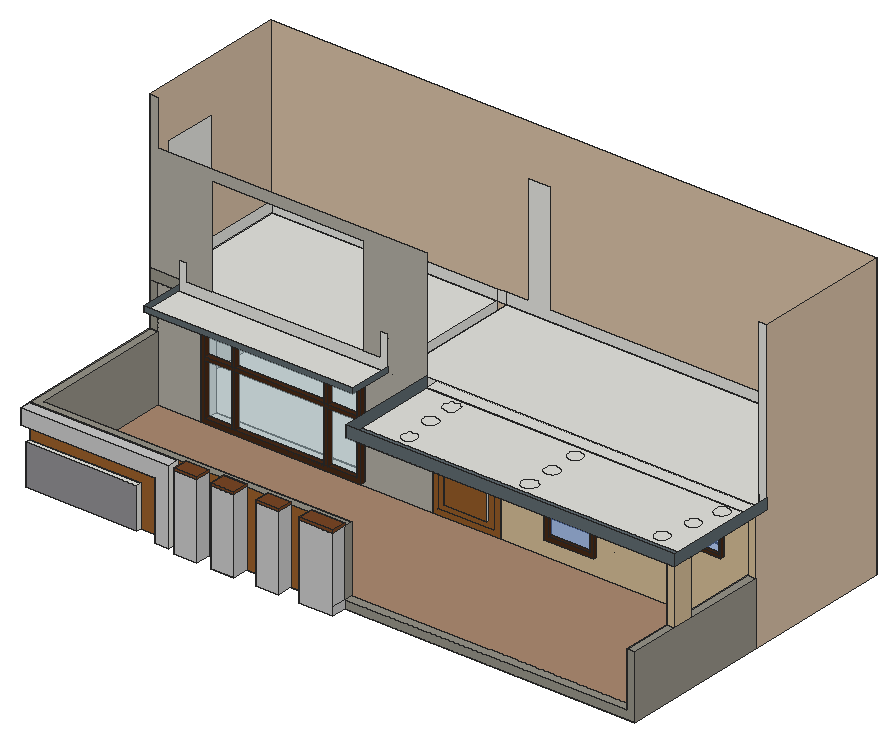
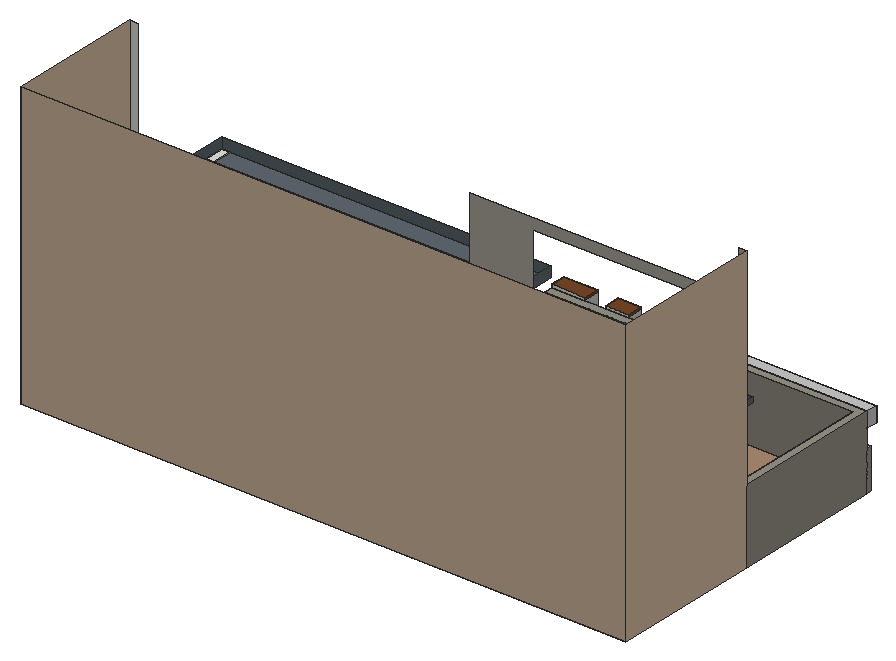
# SketchUp Ruby script. Lengths in inches.
U = 1.inch
M = Sketchup.active_model
def pt(a) = Geom::Point3d.new(a.map { |v| v * U })
def face(e, loops, mat)
  f = e.add_face(loops[0].map { |a| pt(a) })
  loops[1..].each { |l| e.add_face(l.map { |a| pt(a) }).erase! }
  f.material = f.back_material = mat if mat
  f
end
# faces: each face lists its corners as indices into pts; further lists are holes
def faces(e, pts, list, mat = nil) = list.each { |f| face(e, (f[0].is_a?(Array) ? f : [f]).map { |l| l.map { |i| pts[i] } }, mat) }
# xy, xz, yz: faces in a plane at the given z, y or x. An outline is a flat list of corners, or four numbers for a rectangle; further outlines are holes
def ring(l) = l.size == 4 ? [[l[0], l[1]], [l[2], l[1]], [l[2], l[3]], [l[0], l[3]]] : l.each_slice(2).to_a
def flat(e, list, mat, &to3) = list.each { |f| face(e, (f[0].is_a?(Array) ? f : [f]).map { |l| ring(l).map { |u, v| to3.(u, v) } }, mat) }
def xy(e, z, list, mat = nil) = flat(e, list, mat) { |x, y| [x, y, z] }
def xz(e, y, list, mat = nil) = flat(e, list, mat) { |x, z| [x, y, z] }
def yz(e, x, list, mat = nil) = flat(e, list, mat) { |y, z| [x, y, z] }
def lines(e, pts, list) = list.each { |a, b| e.add_line(pt(pts[a]), pt(pts[b])) }
# prism: a flat outline (further loops are holes) pulled along v
def prism(e, loops, v, mat = nil)
  f = face(e, loops, mat); d = Geom::Vector3d.new(v.map { |x| x * U })
  f.pushpull(f.normal.samedirection?(d) ? d.length : -d.length)
end
def box(e, o, s, mat = nil) = prism(e, [[o, [o[0] + s[0], o[1], o[2]], [o[0] + s[0], o[1] + s[1], o[2]], [o[0], o[1] + s[1], o[2]]]], [0, 0, s[2]], mat)
def at(x, y, z, deg = 0) = Geom::Transformation.translation(pt([x, y, z])) * Geom::Transformation.rotation(ORIGIN, Z_AXIS, deg.degrees)
def axes(o, x, y, z) = Geom::Transformation.new([*x, 0, *y, 0, *z, 0, *pt(o).to_a, 1])
def part(name) = M.definitions.add(name)
# library, detail: a bought-in or finely detailed component or shape, given as its bounding box
def library(name, o, s) = part(name).tap { |d| box(d.entities, o, s) }
def detail(e, o, s) = box(e.add_group.entities, o, s)
def put(e, d, t, mat = nil) = e.add_instance(d, t).tap { |i| i.material = mat if mat }
def group(e, t, mat = nil) = e.add_group.tap { |g| g.transformation = t; g.material = mat if mat }.entities
root = M.entities
M.materials.add("[Brick Colored Blue]").color = [144, 143, 146]
M.materials.add("[Cladding Stucco White]").color = [200, 200, 200]
M.materials.add("[Formica Beige]").color = [211, 187, 149]
M.materials.add("[Formica Graystone]").color = [149, 146, 135]
M.materials.add("[Formica Laminate Light]").color = [213, 189, 164]
M.materials.add("[Formica Speckled Grey]").color = [94, 105, 111]
M.materials.add("[Rough Square Concrete Block]").color = [175, 171, 161]
M.materials.add("[Tile Veriegated Stone]").color = [171, 137, 112]
M.materials.add("[Translucent Glass Blue]").color = [100, 149, 237]
M.materials["[Translucent Glass Blue]"].alpha = 0.5
M.materials.add("[Translucent Glass Safety]").color = [204, 235, 244]
M.materials["[Translucent Glass Safety]"].alpha = 0.5
M.materials.add("[Wood Floor Dark]").color = [153, 94, 42]
M.materials.add("[Wood Floor Parquet]").color = [145, 89, 39]
M.materials.add("[Wood Veneer 01]").color = [71, 41, 22]
M.materials.add("[Wood Veneer 01]1").color = [120, 70, 37]
xy(root,0,[[171.65,0,196.76,16.6875],[212.28,0,237.39,16.6875],[260.72,0,285.83,16.6875],[308.45,0,345.33,16.6875],[147.5625,4.3125,162.06,16.6875],
  [0,11.1875,122.3125,16.6875],[0,16.6875,662.71,346.49]])
xy(root,9,[[345.12,0,345.33,16.6875],[309.15,181.59,383.59,196.8125],[9,196.8125,254.94,337.49],[265.25,196.8125,653.71,337.49]])
xy(root,9,[[345.12,16.6875,653.71,25.6875]],"[Formica Graystone]")
xy(root,9,[[9,25.6875,653.71,181.59]],"[Tile Veriegated Stone]")
xy(root,13.06,[[60.26,175.9,235.33,181.59],[60.26,181.59,235.33,196.8125]])
xy(root,17.72,[[64.93,175.9,94.04,181.59],[97.07,175.9,195.15,181.59],[198.84,175.9,230.66,181.59]],"[Wood Veneer 01]")
xy(root,22.49,[[322.64,179.65,370.1,181.59]])
xy(root,28,[[434.23,178.03,488.23,181.59]])
xy(root,32.48,[[438.71,178.03,483.74,181.59]],"[Wood Veneer 01]")
xy(root,44.5,[[0,11.1875,122.3125,16.6875]])
xy(root,64.29,[[0,4.3125,147.5625,16.6875]])
xy(root,68.64,[[653.71,16.6875,662.71,70.96],[653.71,92.91,662.71,181.59]],"[Formica Graystone]")
xy(root,74.8,[[64.93,175.9,94.04,181.59],[97.07,175.9,195.15,181.59],[198.84,175.9,230.66,181.59]])
xy(root,77.28,[[593.34,178.34,627.53,181.59],[593.34,181.59,627.53,196.8125]])
xy(root,78.66,[[64.93,175.9,94.04,181.59],[97.07,175.9,195.15,181.59],[198.84,175.9,230.66,181.59]],"[Wood Veneer 01]")
xy(root,80.01,[[596.07,178.34,624.8,181.59]],"[Wood Veneer 01]")
xy(root,81,[[171.65,0,196.76,16.6875],[212.28,0,237.39,16.6875],[260.72,0,285.83,16.6875],[308.45,0,345.12,16.6875]])
xy(root,81,[[0,4.3125,162.06,16.6875]],"[Cladding Stucco White]")
xy(root,81,[[0,16.6875,345.12,16.6875,345.12,25.6875,9,25.6875,9,181.59,0,181.59]],"[Formica Graystone]")
xy(root,84.0625,[[171.65,0,196.76,16.6875],[212.28,0,237.39,16.6875],[260.72,0,285.83,16.6875],[308.45,0,345.12,16.6875]],"[Wood Veneer 01]1")
xy(root,99.7,[[322.64,179.65,370.1,181.59]])
xy(root,102.27,[[64.93,175.9,94.04,181.59],[97.07,175.9,195.15,181.59],[198.84,175.9,230.66,181.59]])
xy(root,103.95,[[438.71,178.03,483.74,181.59]])
xy(root,105.18,[[596.07,178.34,624.8,181.59]],"[Wood Veneer 01]")
xy(root,106.93,[[60.26,181.59,235.33,196.8125]])
xy(root,106.93,[[60.26,175.9,235.33,181.59]],"[Wood Veneer 01]")
xy(root,107.9,[[593.34,181.59,627.53,196.8125]])
xy(root,107.9,[[593.34,178.34,627.53,181.59]],"[Wood Veneer 01]")
xy(root,108.43,[[434.23,178.03,488.23,181.59]],"[Wood Veneer 01]")
xy(root,113.1875,[[309.15,181.59,383.59,196.8125]])
xy(root,129,[[653.71,70.96,662.71,92.91],[[302.6,92.91,662.71,181.59],[340.27,160.35,342.4375,160.63,344.46,161.47,346.19,162.8,347.52,164.54,348.36,166.56,348.64,168.72,348.36,170.89,347.52,172.91,346.19,174.65,344.46,175.98,342.4375,176.8125,340.27,177.1,338.1,176.8125,336.08,175.98,334.35,174.65,333.02,172.91,332.18,170.89,331.89,168.72,332.18,166.56,333.02,164.54,334.35,162.8,336.08,161.47,338.1,160.63],[344.77,97.13,346.94,97.42,348.95,98.26,350.6875,99.59,352.02,101.32,352.86,103.34,353.14,105.51,352.86,107.68,352.02,109.7,350.6875,111.43,348.95,112.76,346.94,113.6,344.77,113.88,342.6,113.6,340.58,112.76,338.85,111.43,337.51,109.7,336.68,107.68,336.39,105.51,336.68,103.34,337.51,101.32,338.85,99.59,340.58,98.26,342.6,97.42],[341.83,130.04,344,130.33,346.02,131.17,347.76,132.5,349.09,134.23,349.92,136.25,350.21,138.42,349.92,140.59,349.09,142.61,347.76,144.34,346.02,145.67,344,146.51,341.83,146.79,339.67,146.51,337.65,145.67,335.91,144.34,334.58,142.61,333.74,140.59,333.46,138.42,333.74,136.25,334.58,134.23,335.91,132.5,337.65,131.17,339.67,130.33],[476.39,97.13,478.56,97.42,480.58,98.26,482.3125,99.59,483.65,101.32,484.48,103.34,484.77,105.51,484.48,107.68,483.65,109.7,482.3125,111.43,480.58,112.76,478.56,113.6,476.39,113.88,474.22,113.6,472.2,112.76,470.47,111.43,469.14,109.7,468.3,107.68,468.02,105.51,468.3,103.34,469.14,101.32,470.47,99.59,472.2,98.26,474.22,97.42],[621.45,97.13,623.62,97.42,625.64,98.26,627.375,99.59,628.71,101.32,629.54,103.34,629.83,105.51,629.54,107.68,628.71,109.7,627.375,111.43,625.64,112.76,623.62,113.6,621.45,113.88,619.29,113.6,617.27,112.76,615.53,111.43,614.2,109.7,613.37,107.68,613.08,105.51,613.37,103.34,614.2,101.32,615.53,99.59,617.27,98.26,619.29,97.42],[634.6,162.26,636.77,162.54,638.79,163.38,640.52,164.71,641.85,166.45,642.6875,168.47,642.97,170.63,642.6875,172.8,641.85,174.82,640.52,176.56,638.79,177.89,636.77,178.72,634.6,179.01,632.43,178.72,630.41,177.89,628.68,176.56,627.34,174.82,626.51,172.8,626.22,170.63,626.51,168.47,627.34,166.45,628.68,164.71,630.41,163.38,632.43,162.54],[628.15,131.36,630.32,131.65,632.34,132.48,634.07,133.8125,635.4,135.55,636.24,137.57,636.53,139.74,636.24,141.9,635.4,143.92,634.07,145.66,632.34,146.99,630.32,147.83,628.15,148.11,625.98,147.83,623.96,146.99,622.23,145.66,620.9,143.92,620.0625,141.9,619.78,139.74,620.0625,137.57,620.9,135.55,622.23,133.8125,623.96,132.48,625.98,131.65],[476.39,159.7,478.56,159.98,480.58,160.82,482.3125,162.15,483.65,163.88,484.48,165.9,484.77,168.07,484.48,170.24,483.65,172.26,482.3125,173.99,480.58,175.32,478.56,176.16,476.39,176.45,474.22,176.16,472.2,175.32,470.47,173.99,469.14,172.26,468.3,170.24,468.02,168.07,468.3,165.9,469.14,163.88,470.47,162.15,472.2,160.82,474.22,159.98],[476.39,127.45,478.56,127.73,480.58,128.57,482.3125,129.9,483.65,131.63,484.48,133.65,484.77,135.82,484.48,137.99,483.65,140.01,482.3125,141.74,480.58,143.07,478.56,143.91,476.39,144.2,474.22,143.91,472.2,143.07,470.47,141.74,469.14,140.01,468.3,137.99,468.02,135.82,468.3,133.65,469.14,131.63,470.47,129.9,472.2,128.57,474.22,127.73]],[344.77,97.13,342.6,97.42,340.58,98.26,338.85,99.59,337.51,101.32,336.68,103.34,336.39,105.51,336.68,107.68,337.51,109.7,338.85,111.43,340.58,112.76,342.6,113.6,344.77,113.88,346.94,113.6,348.95,112.76,350.6875,111.43,352.02,109.7,352.86,107.68,353.14,105.51,352.86,103.34,352.02,101.32,350.6875,99.59,348.95,98.26,346.94,97.42],[476.39,97.13,474.22,97.42,472.2,98.26,470.47,99.59,469.14,101.32,468.3,103.34,468.02,105.51,468.3,107.68,469.14,109.7,470.47,111.43,472.2,112.76,474.22,113.6,476.39,113.88,478.56,113.6,480.58,112.76,482.3125,111.43,483.65,109.7,484.48,107.68,484.77,105.51,484.48,103.34,483.65,101.32,482.3125,99.59,480.58,98.26,478.56,97.42],[621.45,97.13,619.29,97.42,617.27,98.26,615.53,99.59,614.2,101.32,613.37,103.34,613.08,105.51,613.37,107.68,614.2,109.7,615.53,111.43,617.27,112.76,619.29,113.6,621.45,113.88,623.62,113.6,625.64,112.76,627.375,111.43,628.71,109.7,629.54,107.68,629.83,105.51,629.54,103.34,628.71,101.32,627.375,99.59,625.64,98.26,623.62,97.42],
  [476.39,127.45,474.22,127.73,472.2,128.57,470.47,129.9,469.14,131.63,468.3,133.65,468.02,135.82,468.3,137.99,469.14,140.01,470.47,141.74,472.2,143.07,474.22,143.91,476.39,144.2,478.56,143.91,480.58,143.07,482.3125,141.74,483.65,140.01,484.48,137.99,484.77,135.82,484.48,133.65,483.65,131.63,482.3125,129.9,480.58,128.57,478.56,127.73],[341.83,130.04,339.67,130.33,337.65,131.17,335.91,132.5,334.58,134.23,333.74,136.25,333.46,138.42,333.74,140.59,334.58,142.61,335.91,144.34,337.65,145.67,339.67,146.51,341.83,146.79,344,146.51,346.02,145.67,347.76,144.34,349.09,142.61,349.92,140.59,350.21,138.42,349.92,136.25,349.09,134.23,347.76,132.5,346.02,131.17,344,130.33],[628.15,131.36,625.98,131.65,623.96,132.48,622.23,133.8125,620.9,135.55,620.0625,137.57,619.78,139.74,620.0625,141.9,620.9,143.92,622.23,145.66,623.96,146.99,625.98,147.83,628.15,148.11,630.32,147.83,632.34,146.99,634.07,145.66,635.4,143.92,636.24,141.9,636.53,139.74,636.24,137.57,635.4,135.55,634.07,133.8125,632.34,132.48,630.32,131.65],[31.69,133.78,254.94,181.59],[254.94,133.78,260.09,181.59],
  [476.39,159.7,474.22,159.98,472.2,160.82,470.47,162.15,469.14,163.88,468.3,165.9,468.02,168.07,468.3,170.24,469.14,172.26,470.47,173.99,472.2,175.32,474.22,176.16,476.39,176.45,478.56,176.16,480.58,175.32,482.3125,173.99,483.65,172.26,484.48,170.24,484.77,168.07,484.48,165.9,483.65,163.88,482.3125,162.15,480.58,160.82,478.56,159.98],[340.27,160.35,338.1,160.63,336.08,161.47,334.35,162.8,333.02,164.54,332.18,166.56,331.89,168.72,332.18,170.89,333.02,172.91,334.35,174.65,336.08,175.98,338.1,176.8125,340.27,177.1,342.4375,176.8125,344.46,175.98,346.19,174.65,347.52,172.91,348.36,170.89,348.64,168.72,348.36,166.56,347.52,164.54,346.19,162.8,344.46,161.47,342.4375,160.63],[634.6,162.26,632.43,162.54,630.41,163.38,628.68,164.71,627.34,166.45,626.51,168.47,626.22,170.63,626.51,172.8,627.34,174.82,628.68,176.56,630.41,177.89,632.43,178.72,634.6,179.01,636.77,178.72,638.79,177.89,640.52,176.56,641.85,174.82,642.6875,172.8,642.97,170.63,642.6875,168.47,641.85,166.45,640.52,164.71,638.79,163.38,636.77,162.54],[9,181.59,254.94,196.8125],[302.6,181.59,662.71,196.8125],
  [9,196.8125,254.94,337.49],[265.25,196.8125,653.71,337.49]])
xy(root,129,[[302.6,70.96,653.71,92.91]],"[Formica Speckled Grey]")
xz(root,0,[[171.65,0,196.76,81],[212.28,0,237.39,81],[260.72,0,285.83,81],[308.45,0,345.33,0,345.33,9,345.12,9,345.12,81,308.45,81]],"[Cladding Stucco White]")
xz(root,0,[[171.65,81,196.76,84.0625],[212.28,81,237.39,84.0625],[260.72,81,285.83,84.0625],[308.45,81,345.12,84.0625]],"[Wood Veneer 01]1")
xz(root,4.3125,[[147.5625,0,162.06,0,162.06,81,0,81,0,64.29,147.5625,64.29]],"[Cladding Stucco White]")
xz(root,11.1875,[[0,0,122.3125,44.5]],"[Brick Colored Blue]")
xz(root,16.6875,[[0,0,122.3125,44.5],[147.5625,0,147.5625,64.29,0,64.29,0,81,162.06,81,162.06,0],[171.65,0,196.76,81],[212.28,0,237.39,81],[260.72,0,285.83,81],
  [308.45,0,308.45,81,345.12,81,345.12,9,345.33,9,345.33,0],[345.12,9,345.33,81],[171.65,81,196.76,84.0625],[212.28,81,237.39,84.0625],[260.72,81,285.83,84.0625],
  [308.45,81,345.12,84.0625]])
xz(root,16.6875,[[345.33,0,662.71,0,662.71,68.64,653.71,68.64,653.71,9,345.33,9]],"[Formica Graystone]")
xz(root,16.6875,[[122.3125,0,147.5625,0,147.5625,64.29,0,64.29,0,44.5,122.3125,44.5],[162.06,0,171.65,81],[196.76,0,212.28,81],[237.39,0,260.72,81],[285.83,0,308.45,81]],"[Wood Floor Dark]")
xz(root,25.6875,[[9,9,345.12,81]],"[Formica Graystone]")
xz(root,70.96,[[653.71,68.64,662.71,129]],"[Formica Beige]")
xz(root,70.96,[[302.6,129,662.71,141]],"[Formica Speckled Grey]")
xz(root,92.91,[[653.71,68.64,662.71,129]],"[Formica Beige]")
xz(root,133.78,[[31.69,129,260.09,135]],"[Formica Speckled Grey]")
xz(root,175.9,[[[60.26,13.06,235.33,106.93],[64.93,17.72,230.66,102.27]],[94.04,17.72,97.07,74.8],[195.15,17.72,198.84,74.8],[64.93,74.8,94.04,78.66],[94.04,74.8,97.07,78.66],
  [97.07,74.8,195.15,78.66],[195.15,74.8,198.84,78.66],[198.84,74.8,230.66,78.66],[94.04,78.66,97.07,102.27],[195.15,78.66,198.84,102.27]],"[Wood Veneer 01]")
xz(root,178.03,[[[434.23,28,488.23,108.43],[438.71,32.48,483.74,103.95]]],"[Wood Veneer 01]")
xz(root,178.34,[[[593.34,77.28,627.53,107.9],[596.07,80.01,624.8,105.18]]],"[Wood Veneer 01]")
xz(root,179.65,[[322.64,22.49,370.1,99.7]],"[Wood Floor Parquet]")
xz(root,181.59,[[0,9,9,81],[31.69,129,31.69,159.5,40.13,159.5,40.13,141,251.69,141,251.69,166.97,260.31,166.97,260.09,141,260.09,129]])
xz(root,181.59,[[[383.59,9,653.71,9,653.71,129,309.15,129,309.15,113.1875,383.59,113.1875],[434.23,28,488.23,108.43],[593.34,77.28,627.53,107.9]],[653.71,68.64,662.71,129]],"[Formica Beige]")
xz(root,181.59,[[0,81,9,129],[0,129,31.69,141]],"[Formica Graystone]")
xz(root,181.59,[[[9,9,309.15,9,309.15,129,302.6,129,302.6,261,9,261,9,310.4375,0,310.4375,0,141,31.69,141,31.69,159.5,40.13,159.5,40.13,141,67.84,141,67.84,249.125,233.77,249.125,233.77,141,251.69,141,251.69,166.97,260.31,166.97,260.09,141,260.09,129,9,129],[60.26,13.06,235.33,106.93]]],"[Rough Square Concrete Block]")
xz(root,181.59,[[438.71,32.48,483.74,103.95],[596.07,80.01,624.8,105.18]],"[Translucent Glass Blue]")
xz(root,181.59,[[64.93,17.72,94.04,74.8],[97.07,17.72,195.15,74.8],[198.84,17.72,230.66,74.8],[64.93,78.66,94.04,102.27],[97.07,78.66,195.15,102.27],
  [198.84,78.66,230.66,102.27]],"[Translucent Glass Safety]")
xz(root,181.59,[[[309.15,9,383.59,113.1875],[315.09,14.9375,377.66,107.25]],[[315.09,14.9375,377.66,107.25],[322.64,22.49,370.1,99.7]]],"[Wood Floor Parquet]")
xz(root,196.8125,[[[9,9,254.94,129],[60.26,13.06,235.33,106.93]],[[265.25,9,265.25,129,653.71,129,653.71,9,383.59,9,383.59,113.1875,309.15,113.1875,309.15,9],[436.38,39.78,508.07,111.47],[593.34,77.28,627.53,107.9]],[653.71,129,662.71,310.4375]])
xz(root,337.49,[[9,9,254.94,129],[265.25,9,653.71,129],[9,129,254.94,141],[254.94,129,265.25,141],[265.25,129,265.25,141,289.99,141,289.99,261,312.93,261,312.93,141,653.71,141,653.71,129]])
xz(root,346.49,[[0,0,662.71,310.4375]],"[Formica Laminate Light]")
yz(root,0,[[4.3125,64.29,16.6875,81]],"[Cladding Stucco White]")
yz(root,0,[[11.1875,0,16.6875,44.5],[16.6875,0,181.59,81]],"[Formica Graystone]")
yz(root,0,[[181.59,0,346.49,310.4375]],"[Formica Laminate Light]")
yz(root,9,[[196.8125,9,337.49,129],[196.8125,129,196.8125,261,253.79,261,253.79,141,337.49,141,337.49,129]])
yz(root,9,[[25.6875,9,181.59,81]],"[Formica Graystone]")
yz(root,31.69,[[133.78,129,181.59,135]],"[Formica Speckled Grey]")
yz(root,60.26,[[175.9,13.06,181.59,106.93],[181.59,13.06,196.8125,106.93]])
yz(root,64.93,[[175.9,17.72,181.59,74.8],[175.9,78.66,181.59,102.27]],"[Wood Veneer 01]")
yz(root,94.04,[[175.9,17.72,181.59,74.8],[175.9,78.66,181.59,102.27]],"[Wood Veneer 01]")
yz(root,97.07,[[175.9,17.72,181.59,74.8],[175.9,78.66,181.59,102.27]],"[Wood Veneer 01]")
yz(root,122.3125,[[11.1875,0,16.6875,44.5]])
yz(root,147.5625,[[4.3125,0,16.6875,64.29]],"[Cladding Stucco White]")
yz(root,162.06,[[4.3125,0,16.6875,81]])
yz(root,171.65,[[0,0,16.6875,81]])
yz(root,171.65,[[0,81,16.6875,84.0625]],"[Wood Veneer 01]1")
yz(root,195.15,[[175.9,17.72,181.59,74.8],[175.9,78.66,181.59,102.27]],"[Wood Veneer 01]")
yz(root,196.76,[[0,0,16.6875,81]],"[Cladding Stucco White]")
yz(root,196.76,[[0,81,16.6875,84.0625]],"[Wood Veneer 01]1")
yz(root,198.84,[[175.9,17.72,181.59,74.8],[175.9,78.66,181.59,102.27]],"[Wood Veneer 01]")
yz(root,212.28,[[0,0,16.6875,81]],"[Cladding Stucco White]")
yz(root,212.28,[[0,81,16.6875,84.0625]],"[Wood Veneer 01]1")
yz(root,230.66,[[175.9,17.72,181.59,74.8],[175.9,78.66,181.59,102.27]],"[Wood Veneer 01]")
yz(root,235.33,[[181.59,13.06,196.8125,106.93]])
yz(root,235.33,[[175.9,13.06,181.59,106.93]],"[Wood Veneer 01]")
yz(root,237.39,[[0,0,16.6875,81]],"[Cladding Stucco White]")
yz(root,237.39,[[0,81,16.6875,84.0625]],"[Wood Veneer 01]1")
yz(root,254.94,[[196.8125,9,337.49,129]])
yz(root,260.09,[[133.78,129,181.59,135]],"[Formica Speckled Grey]")
yz(root,260.72,[[0,0,16.6875,81]],"[Cladding Stucco White]")
yz(root,260.72,[[0,81,16.6875,84.0625]],"[Wood Veneer 01]1")
yz(root,265.25,[[196.8125,9,337.49,129]])
yz(root,285.83,[[0,0,16.6875,81]],"[Cladding Stucco White]")
yz(root,285.83,[[0,81,16.6875,84.0625]],"[Wood Veneer 01]1")
yz(root,302.6,[[70.96,129,181.59,141]],"[Formica Speckled Grey]")
yz(root,308.45,[[0,0,16.6875,81]],"[Cladding Stucco White]")
yz(root,308.45,[[0,81,16.6875,84.0625]],"[Wood Veneer 01]1")
yz(root,309.15,[[181.59,9,196.8125,113.1875]])
yz(root,322.64,[[179.65,22.49,181.59,99.7]])
yz(root,345.12,[[0,9,16.6875,81]],"[Cladding Stucco White]")
yz(root,345.12,[[16.6875,9,25.6875,81]],"[Formica Graystone]")
yz(root,345.12,[[0,81,16.6875,84.0625]],"[Wood Veneer 01]1")
yz(root,345.33,[[0,0,16.6875,9]],"[Cladding Stucco White]")
yz(root,370.1,[[179.65,22.49,181.59,99.7]])
yz(root,383.59,[[181.59,9,196.8125,113.1875]])
yz(root,434.23,[[178.03,28,181.59,108.43]],"[Wood Veneer 01]")
yz(root,438.71,[[178.03,32.48,181.59,103.95]],"[Wood Veneer 01]")
yz(root,483.74,[[178.03,32.48,181.59,103.95]],"[Wood Veneer 01]")
yz(root,488.23,[[178.03,28,181.59,108.43]],"[Wood Veneer 01]")
yz(root,593.34,[[181.59,77.28,196.8125,107.9]])
yz(root,593.34,[[178.34,77.28,181.59,107.9]],"[Wood Veneer 01]")
yz(root,596.07,[[178.34,80.01,181.59,105.18]],"[Wood Veneer 01]")
yz(root,624.8,[[178.34,80.01,181.59,105.18]],"[Wood Veneer 01]")
yz(root,627.53,[[181.59,77.28,196.8125,107.9]])
yz(root,627.53,[[178.34,77.28,181.59,107.9]],"[Wood Veneer 01]")
yz(root,653.71,[[196.8125,9,337.49,129],[196.8125,129,337.49,141]])
yz(root,653.71,[[70.96,9,92.91,129]],"[Formica Beige]")
yz(root,653.71,[[16.6875,9,25.6875,68.64],[25.6875,9,70.96,68.64],[92.91,9,181.59,68.64]],"[Formica Graystone]")
yz(root,662.71,[[70.96,68.64,92.91,129]],"[Formica Beige]")
yz(root,662.71,[[16.6875,0,181.59,68.64]],"[Formica Graystone]")
yz(root,662.71,[[181.59,0,346.49,0,346.49,310.4375,196.8125,310.4375,196.8125,129,181.59,129]],"[Formica Laminate Light]")
yz(root,662.71,[[70.96,129,196.8125,141]],"[Formica Speckled Grey]")
p = [[265.25,181.59,129],[265.25,196.8125,129],[436.38,181.59,111.47],[436.38,196.8125,111.47],[508.07,181.59,111.47],[508.07,196.8125,111.47],
  [508.07,181.59,39.78],[508.07,196.8125,39.78]]
lines(root,p,[[0,1],[2,3],[4,5],[6,7]])
